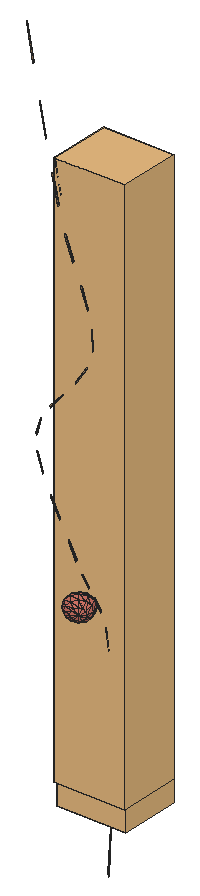
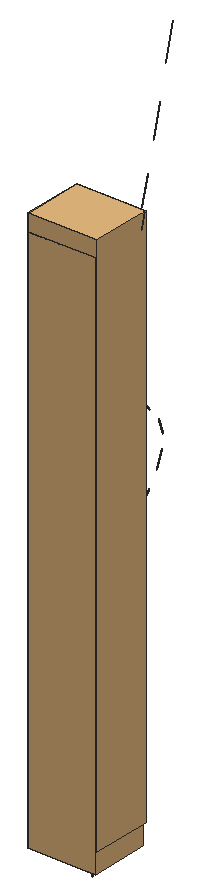
# SketchUp Ruby script. Lengths in inches.
U = 1.inch
M = Sketchup.active_model
def pt(a) = Geom::Point3d.new(a.map { |v| v * U })
def face(e, loops, mat)
  f = e.add_face(loops[0].map { |a| pt(a) })
  loops[1..].each { |l| e.add_face(l.map { |a| pt(a) }).erase! }
  f.material = f.back_material = mat if mat
  f
end
# faces: each face lists its corners as indices into pts; further lists are holes
def faces(e, pts, list, mat = nil) = list.each { |f| face(e, (f[0].is_a?(Array) ? f : [f]).map { |l| l.map { |i| pts[i] } }, mat) }
# xy, xz, yz: faces in a plane at the given z, y or x. An outline is a flat list of corners, or four numbers for a rectangle; further outlines are holes
def ring(l) = l.size == 4 ? [[l[0], l[1]], [l[2], l[1]], [l[2], l[3]], [l[0], l[3]]] : l.each_slice(2).to_a
def flat(e, list, mat, &to3) = list.each { |f| face(e, (f[0].is_a?(Array) ? f : [f]).map { |l| ring(l).map { |u, v| to3.(u, v) } }, mat) }
def xy(e, z, list, mat = nil) = flat(e, list, mat) { |x, y| [x, y, z] }
def xz(e, y, list, mat = nil) = flat(e, list, mat) { |x, z| [x, y, z] }
def yz(e, x, list, mat = nil) = flat(e, list, mat) { |y, z| [x, y, z] }
def lines(e, pts, list) = list.each { |a, b| e.add_line(pt(pts[a]), pt(pts[b])) }
# prism: a flat outline (further loops are holes) pulled along v
def prism(e, loops, v, mat = nil)
  f = face(e, loops, mat); d = Geom::Vector3d.new(v.map { |x| x * U })
  f.pushpull(f.normal.samedirection?(d) ? d.length : -d.length)
end
def box(e, o, s, mat = nil) = prism(e, [[o, [o[0] + s[0], o[1], o[2]], [o[0] + s[0], o[1] + s[1], o[2]], [o[0], o[1] + s[1], o[2]]]], [0, 0, s[2]], mat)
def at(x, y, z, deg = 0) = Geom::Transformation.translation(pt([x, y, z])) * Geom::Transformation.rotation(ORIGIN, Z_AXIS, deg.degrees)
def axes(o, x, y, z) = Geom::Transformation.new([*x, 0, *y, 0, *z, 0, *pt(o).to_a, 1])
def part(name) = M.definitions.add(name)
# library, detail: a bought-in or finely detailed component or shape, given as its bounding box
def library(name, o, s) = part(name).tap { |d| box(d.entities, o, s) }
def detail(e, o, s) = box(e.add_group.entities, o, s)
def put(e, d, t, mat = nil) = e.add_instance(d, t).tap { |i| i.material = mat if mat }
def group(e, t, mat = nil) = e.add_group.tap { |g| g.transformation = t; g.material = mat if mat }.entities
root = M.entities
M.materials.add("green").color = [174, 139, 102]
M.materials.add("vio").color = [206, 114, 100]
c1 = part("3DGeom~157_Defintion")
p = [[36.26,422.52,-32.42],[38.24,377.08,-31.875],[36.84,377.08,-32.625],[36.48,335.72,-32.39],[36.5,298.41,-30.99],[35.18,298.44,-31.7],
  [37.84,335.71,-31.66],[37.69,422.54,-31.65],[32.26,525.68,-30.66],[36.2,472.09,-30.97],[34.73,472.06,-31.76],[33.77,525.72,-29.85],
  [38.91,422.55,-30.49],[40.28,377.08,-29.35],[39.43,377.08,-30.75],[32.92,265.24,-30.5625],[30.44,237.94,-28.41],[29.19,238.08,-29.09],
  [34.2,265.18,-29.87],[39,335.7,-30.56],[38.43,298.38,-28.59],[37.62,298.39,-29.92],[39,335.7,-30.56],[39.83,335.69,-29.19],
  [38.91,422.55,-30.49],[39.79,422.55,-29.05],[35.05,525.75,-28.63],[38.35,472.11,-28.31],[37.45,472.11,-29.79],[35.3,265.14,-28.83],
  [32.28,237.79,-26.11],[31.51,237.83,-27.38],[35.3,265.14,-28.83],[36.08,265.13,-27.54],[35.05,525.75,-28.63],[35.97,525.76,-27.12],
  [23.82,217.46,-27.21],[18.65,200.68,-24.19],[17.48,200.96,-24.87],[25.03,217.22,-26.53],[26.07,217.0625,-25.51],[20.4,200.41,-21.9375],
  [19.66,200.49,-23.18],[26.07,217.0625,-25.51],[26.82,216.99,-24.25],[10.9,186.23,-22.05],[5.93,170.61,-18.08],[4.76,170.8,-18.73],
  [12.06,185.96,-21.38],[13.07,185.79,-20.39],[7.7,170.5,-15.93],[6.95,170.51,-17.12],[13.07,185.79,-20.39],[13.8,185.74,-19.17],
  [20.05,-83.49,-19.57],[20.36,-107.02,-19.07],[19.4,-106.97,-19.5],[21.05,-83.47,-19.125],[21.92,-83.48,-18.41],[21.84,-107.05,-17.47],
  [21.21,-107.04,-18.37],[21.92,-83.48,-18.41],[22.57,-83.5,-17.49],[15.89,-132.25,-16.89],[11.4,-159.71,-12.15],[10.49,-159.62,-12.57],
  [16.82,-132.33,-16.46],[17.65,-132.37,-15.78],[12.79,-159.74,-10.65],[12.19,-159.75,-11.49],[17.65,-132.37,-15.78],[18.26,-132.36,-14.91],
  [8.68,-47.13,-7.48],[17.3,-62.98,-14.9375],[16.31,-63.1,-15.41],[9.65,-46.9375,-6.96],[-0.37,152.09,-14.84],[-4.1,128.9,-8.55],
  [-5.27,128.96,-9.15],[0.82,152,-14.22],[10.53,-46.89,-6.21],[18.84,-63.04,-13.28],[18.18,-62.96,-14.21],[10.53,-46.89,-6.21],
  [11.23,-47.01,-5.28],[1.84,151.98,-13.29],[-2.34,129.04,-6.52],[-3.09,128.93,-7.65],[1.84,151.98,-13.29],[2.59,152.03,-12.12],
  [4.13,-189.34,-7.37],[-1.4,-221.72,-1.7],[-2.26,-221.65,-2.09],[5.01,-189.42,-6.97],[5.79,-189.46,-6.32],[-0.09,-221.74,-0.28],
  [-0.65,-221.75,-1.08],[5.79,-189.46,-6.32],[6.37,-189.45,-5.5],[-10.47,103.92,-1.64],[-14.15,78.09,6.94],[-15.28,78.11,6.38],
  [-9.3125,103.88,-1.06],[-8.3125,103.93,-0.18],[-12.43,78.3,8.88],[-13.16,78.16,7.8],[-8.3125,103.93,-0.18],[-7.57,104.07,0.93],
  [-9.84,-21.39,10.9375],[0.27,-33.63,2.53],[-0.69,-33.86,1.98],[-7.77,-256.8,2.46],[-11.81,-294.96,6.87],[-12.6,-294.92,6.51],
  [-6.94,-256.85,2.84],[-8.85,-21.17,11.49],[-7.96,-21.11,12.28],[1.87,-33.69,4.24],[1.16,-33.57,3.31],[-6.21,-256.87,3.44],
  [-10.59,-294.97,8.17],[-11.11,-294.98,7.4375],[-6.21,-256.87,3.44],[-5.66,-256.86,4.21],[-7.96,-21.11,12.28],[-7.25,-21.21,13.24],
  [-17.49,-335.72,10.65],[-21.71,-379.24,15.19],[-22.42,-379.2,14.875],[-16.73,-335.76,10.98],[-16.07,-335.78,11.53],[-20.62,-379.24,16.37],
  [-21.08,-379.25,15.71],[-16.07,-335.78,11.53],[-15.58,-335.77,12.22],[-19.05,52.72,13.59],[-20.01,29.02,19.21],[-21.11,28.99,18.68],
  [-17.94,52.72,14.13],[-16.97,52.79,14.98],[-18.37,29.18,21.08],[-19.0625,29.08,20.03],[-16.97,52.79,14.98],[-16.26,52.93,16.03],
  [-20.8125,8.25,20.38],[-15.98,-7.82,18.1],[-17.02,-7.99,17.57],[-19.74,8.3125,20.9],[-18.81,8.36,21.71],[-14.38,-7.82,19.9],
  [-15.07,-7.76,18.9],[-27.41,-425.36,19.19],[-31.82,-474.23,23.89],[-32.45,-474.2,23.61],[-26.74,-425.39,19.5],[-18.81,8.36,21.71],
  [-18.13,8.38,22.74],[-26.15,-425.41,19.98],[-30.85,-474.24,24.93],[-31.27,-474.24,24.35],[-26.15,-425.41,19.98],[-25.71,-425.4,20.6]]
faces(c1.entities,p,[[0,1,2],[3,4,5],[3,6,4],[0,7,1],[8,9,10],[8,11,9],[12,13,14],[15,16,17],
  [15,18,16],[19,20,21],[22,23,20],[24,25,13],[26,27,28],[29,30,31],[32,33,30],[34,35,27],
  [36,37,38],[36,39,37],[40,41,42],[43,44,41],[45,46,47],[45,48,46],[49,50,51],[52,53,50],
  [54,55,56],[54,57,55],[58,59,60],[61,62,59],[63,64,65],[63,66,64],[67,68,69],[70,71,68],
  [72,73,74],[72,75,73],[76,77,78],[76,79,77],[80,81,82],[83,84,81],[85,86,87],[88,89,86],
  [90,91,92],[90,93,91],[94,95,96],[97,98,95],[99,100,101],[99,102,100],[103,104,105],[106,107,104],
  [108,109,110],[111,112,113],[111,114,112],[108,115,109],[116,117,118],[119,120,121],[122,123,120],[124,125,117],
  [126,127,128],[126,129,127],[130,131,132],[133,134,131],[135,136,137],[135,138,136],[139,140,141],[142,143,140],
  [144,145,146],[144,147,145],[148,149,150],[151,152,153],[151,154,152],[155,156,149],[157,158,159],[160,161,158]],"green")
c2 = part("3DGeom~246_Defintion")
p = [[52.16,0,-500],[255.625,-213.37,-352.41],[17.91,-184.79,-452.79],[295.17,0,-406.93],[-204.83,0,-459.09],[-224.6,106.69,-431.83],
  [17.91,184.79,-452.79],[-224.6,-106.6875,-431.83],[-406.93,0,-295.17],[-406.93,0,-295.17],[147.59,-369.57,-203.47],[-75.65,-320.06,-323.79],
  [147.59,-369.57,-203.47],[-75.65,-320.06,-323.79],[255.625,213.37,-352.41],[-278.62,184.79,-357.36],[-75.65,320.06,-323.79],[-75.65,-320.06,-323.79],
  [-278.62,-184.79,-357.36],[-278.62,-184.79,-357.36],[-406.93,0,-295.17],[-406.93,0,-295.17],[295.17,0,-406.93],[424.85,-184.79,-157.61],
  [255.625,-213.37,-352.41],[295.17,0,-406.93],[459.09,0,-204.83],[255.625,213.37,-352.41],[295.17,0,-406.93],[-278.62,-184.79,-357.36],
  [-203.47,-369.57,-147.59],[-352.41,-213.37,-255.625],[-278.62,-184.79,-357.36],[-75.65,-320.06,-323.79],[-278.62,-184.79,-357.36],[-352.41,-213.37,-255.625],
  [-406.93,0,-295.17],[-352.41,213.37,-255.625],[-278.62,184.79,-357.36],[-352.41,213.37,-255.625],[-75.65,320.06,-323.79],[-278.62,184.79,-357.36],
  [255.625,-213.37,-352.41],[331.28,-320.06,-28.62],[147.59,-369.57,-203.47],[255.625,-213.37,-352.41],[331.28,-320.06,-28.62],[255.625,213.37,-352.41],
  [424.85,184.79,-157.61],[147.59,369.57,-203.47],[255.625,213.37,-352.41],[147.59,369.57,-203.47],[0,-426.74,0],[147.59,-369.57,-203.47],
  [-352.41,213.37,-255.625],[-203.47,369.57,-147.59],[-75.65,320.06,-323.79],[147.59,369.57,-203.47],[-75.65,320.06,-323.79],[-426.21,-184.79,-153.89],
  [-480.23,-106.6875,-79.42],[-500,0,-52.16],[-480.23,106.6875,-79.42],[-426.21,184.78,-153.89],[-203.47,-369.57,-147.59],[-331.28,-320.06,28.62],
  [-203.47,369.57,-147.59],[480.23,-106.69,79.42],[500,0,52.16],[203.47,-369.57,147.59],[331.28,-320.06,-28.62],[147.59,369.57,-203.47],
  [331.28,320.06,-28.62],[0,426.74,0],[331.28,320.06,-28.62],[147.59,369.57,-203.47],[147.59,369.57,-203.47],[426.21,-184.78,153.89],
  [331.28,-320.06,-28.62],[480.23,106.6875,79.42],[-424.85,-184.78,157.61],[-331.28,320.06,28.62],[-203.47,369.57,-147.59],[-147.59,-369.57,203.47],
  [-147.59,-369.57,203.47],[-331.28,-320.06,28.62],[-331.28,320.06,28.62],[-459.09,0,204.83],[-424.85,184.79,157.61],[331.28,-320.06,-28.62],
  [352.41,-213.37,255.625],[203.47,-369.57,147.59],[331.28,-320.06,-28.62],[426.21,184.79,153.89],[203.47,369.57,147.59],[203.47,369.57,147.59],
  [331.28,320.06,-28.62],[75.65,-320.06,323.79],[-147.59,-369.57,203.47],[75.65,-320.06,323.79],[-331.28,320.06,28.62],[-147.59,369.57,203.47],
  [-147.59,-369.57,203.47],[-255.625,-213.37,352.41],[-147.59,369.57,203.47],[406.93,0,295.17],[278.62,-184.79,357.36],[75.65,-320.06,323.79],
  [352.41,-213.37,255.625],[278.62,-184.79,357.36],[203.47,369.57,147.59],[352.41,213.37,255.625],[75.65,320.06,323.79],[352.41,213.37,255.625],
  [-295.17,0,406.93],[-255.625,213.37,352.41],[-147.59,369.57,203.47],[-147.59,-369.57,203.47],[-17.91,-184.79,452.79],[-255.625,-213.37,352.41],
  [-147.59,-369.57,203.47],[75.65,-320.06,323.79],[-255.625,213.37,352.41],[75.65,320.06,323.79],[-147.59,369.57,203.47],[278.62,-184.79,357.36],
  [278.62,184.79,357.36],[278.62,184.79,357.36],[352.41,213.37,255.625],[224.6,-106.69,431.83],[278.62,-184.79,357.36],[406.93,0,295.17],
  [204.83,0,459.09],[406.93,0,295.17],[224.6,106.6875,431.83],[406.93,0,295.17],[278.62,184.79,357.36],[406.93,0,295.17],
  [-255.625,213.37,352.41],[-17.91,184.79,452.79],[75.65,320.06,323.79],[278.62,184.79,357.36],[75.65,320.06,323.79],[-255.625,-213.37,352.41],
  [-52.16,0,500],[-295.17,0,406.93],[-255.625,-213.37,352.41],[-295.17,0,406.93],[-255.625,213.37,352.41],[278.62,184.79,357.36],
  [-295.17,0,406.93]]
faces(c2.entities,p,[[0,1,2],[0,3,1],[4,0,2],[5,6,0],[5,0,4],[6,3,0],[4,2,7],[4,7,8],
  [5,4,9],[2,10,11],[2,1,12],[7,2,13],[6,14,3],[15,6,5],[15,16,6],[16,14,6],
  [7,17,18],[7,19,20],[15,5,21],[22,23,24],[25,26,23],[27,26,28],[29,30,31],[32,33,30],
  [34,35,36],[37,38,36],[39,40,41],[42,43,44],[45,23,46],[47,48,26],[49,48,50],[16,51,14],
  [33,52,30],[33,53,52],[54,55,56],[55,57,58],[35,59,36],[59,60,36],[60,61,36],[61,62,36],
  [62,63,36],[63,37,36],[35,64,65],[35,65,59],[63,66,37],[26,67,23],[26,68,67],[48,68,26],
  [53,69,52],[53,70,69],[71,72,48],[73,74,75],[55,73,76],[23,77,78],[23,67,77],[48,79,68],
  [72,79,48],[59,65,80],[59,80,60],[62,81,63],[63,81,82],[30,52,83],[30,84,85],[86,73,55],
  [60,80,87],[60,87,61],[61,88,62],[62,88,81],[61,87,88],[89,90,91],[92,77,90],[72,93,79],
  [94,93,72],[73,95,96],[52,97,98],[52,69,99],[100,101,73],[101,95,73],[65,102,103],[65,103,80],
  [88,104,81],[67,68,105],[68,79,105],[77,67,105],[79,93,105],[69,106,107],[69,108,109],[110,111,93],
  [112,113,95],[101,112,95],[90,77,105],[93,111,105],[80,103,114],[80,114,87],[87,115,88],[88,115,116],
  [117,118,119],[120,121,118],[122,123,124],[87,114,115],[125,90,105],[111,126,105],[112,127,128],[129,130,131],
  [132,129,133],[134,132,135],[136,134,137],[121,129,118],[121,130,129],[138,139,140],[139,141,142],[143,144,145],
  [146,118,144],[147,139,148],[139,134,149],[150,144,139],[118,129,132],[144,132,134],[144,134,139],[118,132,144]],"vio")
c3 = part("3DGeom~39_Defintion")
p = [[35.12,-55.5,-54.41],[34.11,-55.53,-54.86],[35.81,-76.47,-55.34],[36.8,-76.41,-54.9],[38.88,-99.33,-54.67],[37.91,-99.4,-55.11],
  [39.32,-123.69,-53.625],[40.28,-123.64,-53.2],[37.08,-24.79,-53.05],[36.07,-24.5,-53.5],[33.89,-37.16,-54.23],[34.93,-37.21,-53.77],
  [44.64,-14.39,-49.98],[39.94,-17.85,-52.2],[40.77,-18.46,-51.8125],[43.83,-13.75,-50.35],[39.93,-148.71,-49.9375],[38.99,-148.72,-50.36],
  [35.86,-173.84,-44.78],[36.78,-173.89,-44.36],[49.18,2.9,-43.4],[46.875,-8.22,-47.77],[47.86,-8.59,-47.26],[48.17,3.01,-43.99],
  [40.94,55.6,-31.2],[39.91,55.54,-31.86],[46.25,23.72,-38.95],[47.26,23.73,-38.32],[29.9,-199.58,-35.34],[29.03,-199.5,-35.76],
  [19.05,-226.47,-23.39],[19.9,-226.57,-22.96],[18.98,142.12,-11.91],[17.89,142.02,-12.62],[29.92,96.01,-22.77],[30.98,96.1,-22.08],
  [8.08,-254.51,-8.72],[7.27,-254.41,-9.13],[-4.99,-283,5.49],[-4.2,-283.09,5.89],[-4.75,238.47,7.76],[-5.91,238.39,7],
  [5.41,190.5,-2.38],[6.54,190.59,-1.65],[-19.28,323.69,21.26],[-20.52,323.65,20.47],[-14.48,282.67,14.58],[-13.28,282.72,15.35],
  [-15.6,-312.05,19.375],[-16.37,-311.96,18.99],[-25.53,-341.05,29.86],[-24.78,-341.11,30.22],[-27.78,403.71,30.46],[-29.08,403.69,29.63],
  [-25.39,363.99,25.48],[-24.12,364.02,26.29],[-31.6,481.16,36.19],[-32.96,481.18,35.32],[-31.61,442.75,32.91],[-30.28,442.76,33.76],
  [-31.87,-370.06,38.59],[-32.6,-370.01,38.24],[-38.75,-399.23,45.4375],[-38.04,-399.28,45.77],[-43.3,-428.76,51.78],[-43.98,-428.72,51.46],
  [-48.3,-458.49,56.3],[-47.64,-458.51,56.62],[-51.06,-488.54,60.27],[-51.7,-488.51,59.97],[-54.18,-518.81,62.46],[-53.57,-518.82,62.75]]
faces(c3.entities,p,[[0,1,2],[0,2,3],[4,5,6],[4,6,7],[8,9,10],[8,10,11],[12,13,14],[12,15,13],
  [16,17,18],[16,18,19],[20,21,22],[20,23,21],[24,25,26],[24,26,27],[28,29,30],[28,30,31],
  [32,33,34],[32,34,35],[36,37,38],[36,38,39],[40,41,42],[40,42,43],[44,45,46],[44,46,47],
  [48,49,50],[48,50,51],[52,53,54],[52,54,55],[56,57,58],[56,58,59],[60,61,62],[60,62,63],
  [64,65,66],[64,66,67],[68,69,70],[68,70,71]],"green")
c4 = part("3DGeom~43_Defintion")
p = [[34.1,-55.53,-54.86],[33.24,-55.55,-55.5625],[34.97,-76.52,-56.03],[34.97,-76.52,-56.03],[35.81,-76.47,-55.34],[37.9,-99.39,-55.1],
  [37.08,-99.46,-55.78],[38.51,-123.75,-54.29],[38.51,-123.75,-54.29],[39.32,-123.6875,-53.625],[36.18,-55.46,-54.25],[35.12,-55.5,-54.41],
  [36.8,-76.4,-54.89],[37.84,-76.34,-54.74],[36.07,-24.5,-53.5],[33.01,-37.11,-54.9375],[33.89,-37.16,-54.22],[35.22,-24.22,-54.2],
  [33.01,-37.11,-54.9375],[39.9,-99.26,-54.51],[38.875,-99.33,-54.67],[40.28,-123.64,-53.2],[41.28,-123.61,-53.04],[38.13,-25.08,-52.89],
  [34.92,-37.21,-53.77],[36.01,-37.26,-53.6],[37.08,-24.79,-53.05],[43.83,-13.75,-50.35],[39.26,-17.27,-52.85],[39.94,-17.85,-52.2],
  [43.19,-13.12,-50.98],[39.26,-17.27,-52.85],[45.52,-14.98,-49.89],[40.76,-18.46,-51.81],[41.65,-19.04,-51.71],[44.63,-14.39,-49.98],
  [38.99,-148.71,-50.36],[38.2,-148.76,-51.01],[35.09,-173.85,-45.42],[35.09,-173.85,-45.42],[35.86,-173.83,-44.78],[40.91,-148.73,-49.78],
  [39.93,-148.7,-49.9375],[36.77,-173.88,-44.35],[37.72,-173.98,-44.18],[48.17,3.01,-43.99],[46.09,-7.82,-48.51],[46.875,-8.22,-47.76],
  [48.17,3.01,-43.99],[47.35,3.18,-44.83],[50.28,2.84,-43.09],[47.85,-8.59,-47.25],[48.92,-8.89,-47.03],[49.18,2.9,-43.39],
  [39.91,55.53,-31.86],[45.4375,23.76,-39.82],[46.25,23.72,-38.95],[39.91,55.53,-31.86],[39.08,55.54,-32.77],[42.07,55.72,-30.83],
  [40.94,55.6,-31.2],[47.26,23.73,-38.3125],[48.36,23.79,-37.97],[29.03,-199.49,-35.76],[28.28,-199.5,-36.39],[18.33,-226.47,-24],
  [18.33,-226.47,-24],[19.05,-226.46,-23.38],[30.81,-199.72,-35.15],[29.9,-199.57,-35.34],[19.9,-226.56,-22.96],[20.77,-226.74,-22.76],
  [17.89,142.02,-12.62],[17.01,142,-13.59],[29.07,96,-23.71],[17.89,142.02,-12.62],[29.92,96.01,-22.77],[20.17,142.27,-11.51],
  [18.98,142.11,-11.91],[30.98,96.09,-22.07],[32.14,96.24,-21.69],[7.27,-254.4,-9.13],[6.56,-254.4,-9.73],[-5.67,-282.99,4.91],
  [-5.67,-282.99,4.91],[-4.99,-282.98,5.49],[8.92,-254.68,-8.52],[8.08,-254.5,-8.72],[-4.2,-283.08,5.89],[-3.38,-283.26,6.08],
  [-5.91,238.375,7],[-6.85,238.36,5.97],[4.51,190.47,-3.39],[-5.91,238.375,7],[5.41,190.49,-2.38],[-3.48,238.6,8.17],
  [-4.75,238.46,7.76],[6.54,190.58,-1.65],[7.77,190.74,-1.24],[-20.52,323.63,20.47],[-21.51,323.64,19.38],[-15.45,282.66,13.52],
  [-20.52,323.63,20.47],[-14.48,282.65,14.58],[-17.93,323.76,21.68],[-19.28,323.68,21.26],[-13.28,282.71,15.35],[-11.96,282.8125,15.77],
  [-16.37,-311.95,18.99],[-17.03,-311.95,18.43],[-26.16,-341.03,29.3125],[-26.16,-341.03,29.3125],[-25.53,-341.03,29.86],[-14.8,-312.18,19.55],
  [-15.6,-312.03,19.375],[-24.78,-341.09,30.22],[-23.99,-341.2,30.375],[-29.08,403.67,29.63],[-30.12,403.6875,28.5],[-26.4,363.98,24.37],
  [-29.08,403.67,29.63],[-25.39,363.97,25.48],[-26.36,403.74,30.9],[-27.78,403.6875,30.46],[-24.12,364,26.29],[-22.73,364.07,26.72],
  [-32.96,481.15,35.32],[-32.67,442.75,31.75],[-31.61,442.73,32.91],[-32.96,481.15,35.32],[-34.05,481.18,34.13],[-30.11,481.14,36.64],
  [-31.6,481.14,36.18],[-30.28,442.73,33.76],[-28.82,442.76,34.2],[-32.6,-369.99,38.23],[-33.21,-369.99,37.71],[-39.34,-399.21,44.93],
  [-39.34,-399.21,44.93],[-38.75,-399.21,45.43],[-31.11,-370.14,38.73],[-31.87,-370.04,38.58],[-38.04,-399.25,45.77],[-37.3,-399.34,45.91],
  [-43.98,-428.7,51.46],[-44.55,-428.7,50.97],[-48.85,-458.46,55.83],[-48.85,-458.46,55.83],[-48.3,-458.46,56.3],[-42.58,-428.8,51.91],
  [-43.3,-428.74,51.78],[-47.64,-458.49,56.61],[-46.95,-458.54,56.74],[-51.7,-488.49,59.97],[-52.23,-488.48,59.51],[-54.6875,-518.78,62.02],
  [-54.6875,-518.78,62.02],[-54.18,-518.78,62.46],[-50.4,-488.55,60.39],[-51.0625,-488.51,60.27],[-53.57,-518.8,62.75],[-52.93,-518.82,62.86]]
faces(c4.entities,p,[[0,1,2],[0,3,4],[5,6,7],[5,8,9],[10,11,12],[10,12,13],[14,15,16],[14,17,18],
  [19,20,21],[19,21,22],[23,24,25],[23,26,24],[27,28,29],[27,30,31],[32,33,34],[32,35,33],
  [36,37,38],[36,39,40],[41,42,43],[41,43,44],[45,46,47],[48,49,46],[50,51,52],[50,53,51],
  [54,55,56],[57,58,55],[59,60,61],[59,61,62],[63,64,65],[63,66,67],[68,69,70],[68,70,71],
  [72,73,74],[75,74,76],[77,78,79],[77,79,80],[81,82,83],[81,84,85],[86,87,88],[86,88,89],
  [90,91,92],[93,92,94],[95,96,97],[95,97,98],[99,100,101],[102,101,103],[104,105,106],[104,106,107],
  [108,109,110],[108,111,112],[113,114,115],[113,115,116],[117,118,119],[120,119,121],[122,123,124],[122,124,125],
  [126,127,128],[129,130,127],[131,132,133],[131,133,134],[135,136,137],[135,138,139],[140,141,142],[140,142,143],
  [144,145,146],[144,147,148],[149,150,151],[149,151,152],[153,154,155],[153,156,157],[158,159,160],[158,160,161]],"green")
c5 = part("3DGeom~38_Defintion")
p = [[36.53,-75.84,-54.49],[35.54,-75.9,-54.93],[37.625,-98.66,-54.7],[38.59,-98.59,-54.27],[34.67,-36.9375,-53.37],[33.64,-36.89,-53.82],
  [33.85,-55.12,-54.46],[34.86,-55.09,-54.01],[39.98,-122.72,-52.8],[39.03,-122.77,-53.23],[38.7,-147.61,-49.99],[40.46,-18.32,-51.43],
  [35.81,-24.32,-53.1],[36.81,-24.61,-52.65],[39.64,-17.72,-51.8125],[39.63,-147.6,-49.57],[47.5,-8.52,-46.91],[43.5,-13.65,-49.98],
  [44.3,-14.29,-49.61],[46.53,-8.16,-47.41],[36.5,-172.59,-44.03],[35.6,-172.55,-44.45],[28.8125,-198.01,-35.5],[29.68,-198.09,-35.07],
  [46.91,23.55,-38.03],[47.81,2.99,-43.67],[48.82,2.875,-43.07],[45.91,23.54,-38.66],[30.75,95.38,-21.91],[29.7,95.3,-22.6],
  [39.61,55.12,-31.625],[40.64,55.18,-30.97],[19.75,-224.88,-22.79],[18.91,-224.79,-23.21],[7.21,-252.52,-9.07],[8.02,-252.62,-8.65],
  [6.49,189.18,-1.63],[5.37,189.08,-2.36],[17.76,140.97,-12.53],[18.84,141.0625,-11.82],[-4.17,-280.99,5.85],[-4.95,-280.89,5.45],
  [-16.25,-309.64,18.85],[-15.49,-309.73,19.23],[-13.18,280.62,15.24],[-14.375,280.56,14.47],[-5.87,236.61,6.95],[-4.71,236.7,7.7],
  [-23.9375,361.3125,26.1],[-25.2,361.28,25.3],[-20.37,321.24,20.31],[-19.14,321.29,21.1],[-30.05,439.46,33.51],[-31.375,439.46,32.67],
  [-28.87,400.6875,29.41],[-27.58,400.7,30.23],[-24.59,-338.57,30],[-25.34,-338.51,29.63],[-32.35,-367.25,37.95],[-31.63,-367.31,38.3],
  [-31.52,515.07,37.46],[-32.9,515.1,36.59],[-32.72,477.6,35.0625],[-31.37,477.58,35.92],[-37.76,-396.3,45.43],[-38.46,-396.26,45.1],
  [-43.65,-425.53,51.08],[-42.98,-425.57,51.4],[-47.29,-455.1,56.19],[-47.9375,-455.07,55.89],[-51.3125,-484.88,59.53],[-50.68,-484.9,59.82]]
faces(c5.entities,p,[[0,1,2],[0,2,3],[4,5,6],[4,6,7],[8,9,10],[11,12,13],[11,14,12],[8,10,15],
  [16,17,18],[16,19,17],[20,21,22],[20,22,23],[24,25,26],[24,27,25],[28,29,30],[28,30,31],
  [32,33,34],[32,34,35],[36,37,38],[36,38,39],[40,41,42],[40,42,43],[44,45,46],[44,46,47],
  [48,49,50],[48,50,51],[52,53,54],[52,54,55],[56,57,58],[56,58,59],[60,61,62],[60,62,63],
  [64,65,66],[64,66,67],[68,69,70],[68,70,71]],"green")
c6 = part("3DGeom~41_Defintion")
p = [[35.54,-75.9,-54.92],[34.7,-75.95,-55.61],[36.8,-98.72,-55.36],[36.8,-98.72,-55.36],[37.62,-98.65,-54.69],[33.64,-36.88,-53.82],
  [32.76,-36.83,-54.53],[33,-55.14,-55.15],[33,-55.14,-55.15],[33.85,-55.12,-54.45],[37.55,-75.77,-54.33],[36.52,-75.83,-54.49],
  [38.59,-98.59,-54.26],[39.6,-98.52,-54.11],[35.74,-36.98,-53.2],[34.66,-36.93,-53.37],[34.86,-55.09,-54.01],[35.91,-55.05,-53.84],
  [39.03,-122.76,-53.22],[38.22,-122.82,-53.88],[37.91,-147.65,-50.63],[39.64,-17.72,-51.81],[34.96,-24.04,-53.8],[35.8,-24.32,-53.1],
  [38.97,-17.14,-52.46],[34.96,-24.04,-53.8],[37.91,-147.65,-50.63],[38.7,-147.6,-49.98],[40.97,-122.6875,-52.65],[39.97,-122.72,-52.8],
  [39.63,-147.59,-49.5625],[41.34,-18.9,-51.33],[36.8,-24.61,-52.65],[37.85,-24.89,-52.5],[40.46,-18.32,-51.42],[40.6,-147.62,-49.41],
  [46.52,-8.16,-47.41],[42.87,-13.02,-50.6],[43.5,-13.65,-49.97],[45.74,-7.77,-48.15],[42.87,-13.02,-50.6],[48.56,-8.83,-46.68],
  [44.3,-14.29,-49.6],[45.18,-14.87,-49.52],[47.5,-8.52,-46.9],[35.6,-172.54,-44.45],[34.83,-172.56,-45.08],[28.07,-198.01,-36.12],
  [45.91,23.54,-38.65],[47,3.16,-44.49],[47.81,2.99,-43.66],[45.91,23.54,-38.65],[45.1,23.59,-39.52],[28.07,-198.01,-36.12],
  [28.8125,-198,-35.5],[37.44,-172.68,-43.85],[36.5,-172.58,-44.02],[29.68,-198.08,-35.07],[30.58,-198.23,-34.88],[48,23.61,-37.69],
  [48.8125,2.875,-43.07],[49.91,2.82,-42.76],[46.91,23.55,-38.03],[29.7,95.29,-22.6],[28.85,95.28,-23.53],[38.79,55.13,-32.53],
  [29.7,95.29,-22.6],[39.61,55.12,-31.625],[31.9,95.53,-21.53],[30.75,95.375,-21.91],[40.64,55.18,-30.96],[41.75,55.31,-30.6],
  [18.91,-224.77,-23.21],[18.19,-224.78,-23.82],[6.52,-252.5,-9.66],[6.52,-252.5,-9.66],[7.21,-252.5,-9.07],[20.61,-225.05,-22.59],
  [19.75,-224.87,-22.79],[8.02,-252.6,-8.65],[8.86,-252.78,-8.46],[5.37,189.07,-2.36],[4.47,189.05,-3.36],[16.88,140.94,-13.49],
  [5.37,189.07,-2.36],[17.75,140.96,-12.53],[7.71,189.32,-1.23],[6.49,189.16,-1.63],[18.84,141.05,-11.82],[20.02,141.21,-11.43],
  [-4.95,-280.875,5.45],[-5.63,-280.875,4.875],[-16.9,-309.625,18.29],[-16.9,-309.625,18.29],[-16.25,-309.62,18.85],[-3.36,-281.15,6.04],
  [-4.17,-280.97,5.85],[-15.49,-309.7,19.23],[-14.375,280.54,14.47],[-15.33,280.55,13.42],[-6.79,236.59,5.92],[-14.375,280.54,14.47],
  [-5.87,236.6,6.95],[-14.69,-309.86,19.4],[-11.87,280.7,15.65],[-13.18,280.6,15.24],[-4.71,236.68,7.7],[-3.45,236.82,8.11],
  [-25.2,361.26,25.29],[-26.2,361.27,24.19],[-21.35,321.23,19.24],[-25.2,361.26,25.29],[-20.37,321.22,20.3125],[-22.5625,361.36,26.52],
  [-23.9375,361.29,26.09],[-19.14,321.26,21.1],[-17.8,321.35,21.52],[-31.37,439.43,32.67],[-32.43,439.45,31.51],[-29.9,400.68,28.28],
  [-31.37,439.43,32.67],[-28.87,400.66,29.41],[-25.34,-338.49,29.63],[-25.97,-338.49,29.09],[-32.96,-367.23,37.43],[-32.96,-367.23,37.43],
  [-32.35,-367.23,37.95],[-23.81,-338.66,30.15],[-24.59,-338.55,29.99],[-31.63,-367.28,38.3],[-30.875,-367.375,38.44],[-28.61,439.46,33.95],
  [-30.05,439.43,33.5],[-27.58,400.68,30.23],[-26.16,400.72,30.67],[-32.9,515.0625,36.59],[-34,515.1,35.38],[-33.79,477.59,33.88],
  [-32.9,515.0625,36.59],[-32.72,477.5625,35.06],[-30,515.01,37.92],[-31.51,515.03,37.46],[-31.36,477.55,35.91],[-29.89,477.55,36.37],
  [-38.46,-396.23,45.09],[-39.05,-396.23,44.59],[-44.22,-425.5,50.59],[-44.22,-425.5,50.59],[-43.65,-425.5,51.07],[-37.03,-396.36,45.57],
  [-37.76,-396.28,45.43],[-42.98,-425.54,51.39],[-42.27,-425.61,51.52],[-47.9375,-455.04,55.88],[-48.48,-455.04,55.41],[-51.84,-484.84,59.07],
  [-51.84,-484.84,59.07],[-51.31,-484.84,59.52],[-46.6,-455.12,56.3125],[-47.28,-455.07,56.19],[-50.68,-484.87,59.82],[-50.02,-484.9,59.9375]]
faces(c6.entities,p,[[0,1,2],[0,3,4],[5,6,7],[5,8,9],[10,11,12],[10,12,13],[14,15,16],[14,16,17],
  [18,19,20],[21,22,23],[21,24,25],[18,26,27],[28,29,30],[31,32,33],[31,34,32],[28,30,35],
  [36,37,38],[36,39,40],[41,42,43],[41,44,42],[45,46,47],[48,49,50],[51,52,49],[45,53,54],
  [55,56,57],[55,57,58],[59,60,61],[59,62,60],[63,64,65],[66,65,67],[68,69,70],[68,70,71],
  [72,73,74],[72,75,76],[77,78,79],[77,79,80],[81,82,83],[84,83,85],[86,87,88],[86,88,89],
  [90,91,92],[90,93,94],[95,96,97],[98,99,100],[101,100,102],[95,97,103],[104,105,106],[104,106,107],
  [108,109,110],[111,110,112],[113,114,115],[113,115,116],[117,118,119],[120,119,121],[122,123,124],[122,125,126],
  [127,128,129],[127,129,130],[131,132,133],[131,133,134],[135,136,137],[138,137,139],[140,141,142],[140,142,143],
  [144,145,146],[144,147,148],[149,150,151],[149,151,152],[153,154,155],[153,156,157],[158,159,160],[158,160,161]],"green")
c7 = library("3DGeom~45_Defintion",[-55.29,-518.75,-62.82],[110.58,1000,125.64])
c8 = library("3DGeom~42_Defintion",[-55.29,-518.75,-62.82],[110.58,1000,125.58])
c9 = library("3DGeom~44_Defintion",[-52.47,-485.07,-62.35],[107.35,1000,122.25])
c10 = library("3DGeom~40_Defintion",[-52.47,-485.07,-62.35],[107.35,1000,122.2])
c11 = library("3DGeom~55_Defintion",[-110.06,-500,-128.16],[220.12,1000,256.32])
c12 = part("3DGeom~56_Defintion")
p = [[97.55,-500,-116.33],[81.6,-498.52,-119.3],[89.92,-499.6,-119.93],[81.6,-498.52,-119.3],[97.55,-500,-116.33],[71.36,-495.57,-107.07],
  [81.6,-498.52,-119.3],[71.36,-495.57,-107.07],[74.8,-497.04,-114.59],[71.36,-495.57,-107.07],[97.55,-500,-116.33],[77.08,-494.09,-91.89],
  [77.08,-494.09,-91.89],[97.55,-500,-116.33],[93.03,-495.57,-88.93],[93.03,-495.57,-88.93],[97.55,-500,-116.33],[103.26,-498.52,-101.15],
  [97.55,-500,-116.33],[102.43,-499.6,-109.46],[103.26,-498.52,-101.15],[71.36,-495.57,-107.07],[77.08,-494.09,-91.89],[72.19,-494.49,-98.77],
  [93.03,-495.57,-88.93],[103.26,-498.52,-101.15],[99.82,-497.04,-93.63],[77.08,-494.09,-91.89],[93.03,-495.57,-88.93],[84.7,-494.49,-88.29],
  [-84.43,500,100.9375],[-92,499.375,97.28],[-100.19,497.67,97.75],[-84.43,500,100.9375],[-100.19,497.67,97.75],[-106.8,495.34,102.24],
  [-84.43,500,100.9375],[-109.09,491.3,117.68],[-104.16,490.68,124.5],[-84.43,500,100.9375],[-104.16,490.68,124.5],[-96.58,491.3,128.16],
  [-84.43,500,100.9375],[-110.06,493.01,109.53],[-109.09,491.3,117.68],[-84.43,500,100.9375],[-96.58,491.3,128.16],[-88.39,493.01,127.68],
  [-84.43,500,100.9375],[-106.8,495.34,102.24],[-110.06,493.01,109.53],[-84.43,500,100.9375],[-88.39,493.01,127.68],[-81.78,495.34,123.2],
  [-84.43,500,100.9375],[-81.78,495.34,123.2],[-78.53,497.67,115.9],[-84.43,500,100.9375],[-78.53,497.67,115.9],[-79.49,499.375,107.75]]
faces(c12.entities,p,[[0,1,2],[3,4,5],[6,7,8],[9,10,11],[12,13,14],[15,16,17],[18,19,20],[21,22,23],
  [24,25,26],[27,28,29],[30,31,32],[33,34,35],[36,37,38],[39,40,41],[42,43,44],[45,46,47],
  [48,49,50],[51,52,53],[54,55,56],[57,58,59]],"green")
put(root,c1,axes([14.3,134.2,35.93],[0,0.01104,0],[0,0,-0.01104],[-0.01104,0,0]),"green")
g1 = group(root,at(15.3125,134.49,26.21))
put(g1,c2,axes([-0.94,-0.125,7.35],[0,0.00039,0],[0,0,-0.00039],[-0.00039,0,0]),"vio")
put(root,c3,axes([14.37,134.99,34.91],[0,0.00798,0],[0,0,-0.00798],[-0.00798,0,0]),"green")
put(root,c4,axes([14.37,134.99,34.91],[0,0.00798,0],[0,0,-0.00798],[-0.00798,0,0]),"green")
put(root,c5,axes([14.37,134.99,34.91],[0,0.00804,0],[0,0,-0.00804],[-0.00804,0,0]),"green")
put(root,c6,axes([14.37,134.99,34.91],[0,0.00804,0],[0,0,-0.00804],[-0.00804,0,0]),"green")
put(root,c7,axes([14.37,134.99,34.91],[0,0.00799,0],[0,0,-0.00799],[-0.00799,0,0]),"green")
put(root,c8,axes([14.37,134.99,34.91],[0,0.00799,0],[0,0,-0.00799],[-0.00799,0,0]),"green")
put(root,c9,axes([14.37,134.99,34.91],[0,0.00805,0],[0,0,-0.00805],[-0.00805,0,0]),"green")
put(root,c10,axes([14.37,134.99,34.91],[0,0.00805,0],[0,0,-0.00805],[-0.00805,0,0]),"green")
g2 = group(root,at(15.3125,134.49,26.21))
put(g2,c11,axes([-0.92,0.53,7.11],[0,0.00091,0],[0,0,-0.00091],[-0.00091,0,0]),"green")
put(g2,c12,axes([-0.92,0.53,7.11],[0,0.00091,0],[0,0,-0.00091],[-0.00091,0,0]),"green")
